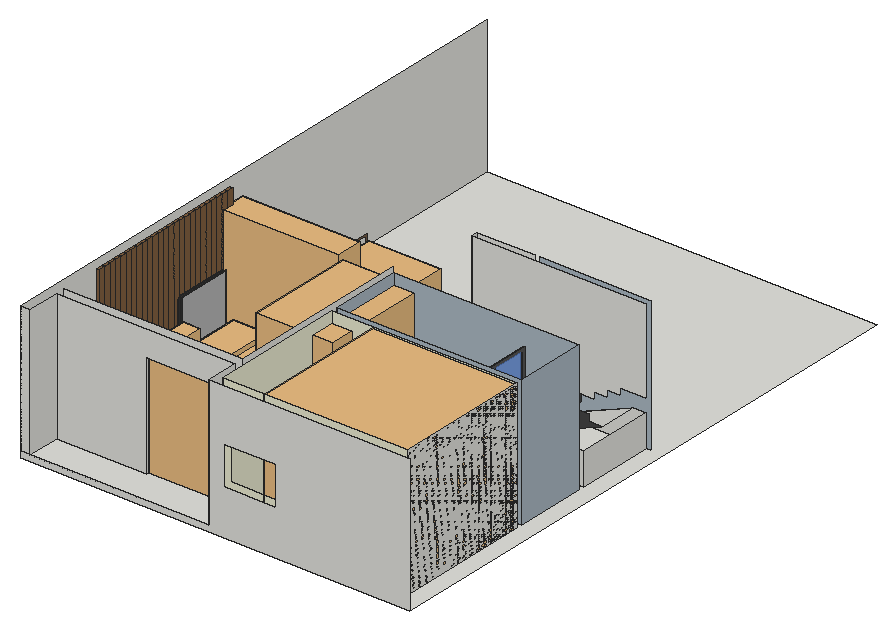
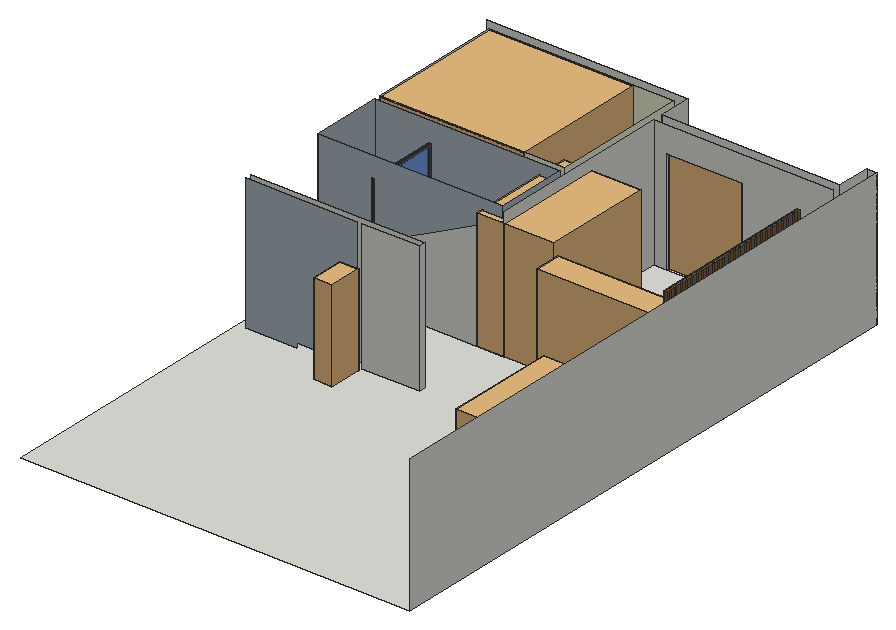
# SketchUp Ruby script. Lengths in inches.
U = 1.inch
M = Sketchup.active_model
def pt(a) = Geom::Point3d.new(a.map { |v| v * U })
def face(e, loops, mat)
  f = e.add_face(loops[0].map { |a| pt(a) })
  loops[1..].each { |l| e.add_face(l.map { |a| pt(a) }).erase! }
  f.material = f.back_material = mat if mat
  f
end
# faces: each face lists its corners as indices into pts; further lists are holes
def faces(e, pts, list, mat = nil) = list.each { |f| face(e, (f[0].is_a?(Array) ? f : [f]).map { |l| l.map { |i| pts[i] } }, mat) }
# xy, xz, yz: faces in a plane at the given z, y or x. An outline is a flat list of corners, or four numbers for a rectangle; further outlines are holes
def ring(l) = l.size == 4 ? [[l[0], l[1]], [l[2], l[1]], [l[2], l[3]], [l[0], l[3]]] : l.each_slice(2).to_a
def flat(e, list, mat, &to3) = list.each { |f| face(e, (f[0].is_a?(Array) ? f : [f]).map { |l| ring(l).map { |u, v| to3.(u, v) } }, mat) }
def xy(e, z, list, mat = nil) = flat(e, list, mat) { |x, y| [x, y, z] }
def xz(e, y, list, mat = nil) = flat(e, list, mat) { |x, z| [x, y, z] }
def yz(e, x, list, mat = nil) = flat(e, list, mat) { |y, z| [x, y, z] }
def lines(e, pts, list) = list.each { |a, b| e.add_line(pt(pts[a]), pt(pts[b])) }
# prism: a flat outline (further loops are holes) pulled along v
def prism(e, loops, v, mat = nil)
  f = face(e, loops, mat); d = Geom::Vector3d.new(v.map { |x| x * U })
  f.pushpull(f.normal.samedirection?(d) ? d.length : -d.length)
end
def box(e, o, s, mat = nil) = prism(e, [[o, [o[0] + s[0], o[1], o[2]], [o[0] + s[0], o[1] + s[1], o[2]], [o[0], o[1] + s[1], o[2]]]], [0, 0, s[2]], mat)
def at(x, y, z, deg = 0) = Geom::Transformation.translation(pt([x, y, z])) * Geom::Transformation.rotation(ORIGIN, Z_AXIS, deg.degrees)
def axes(o, x, y, z) = Geom::Transformation.new([*x, 0, *y, 0, *z, 0, *pt(o).to_a, 1])
def part(name) = M.definitions.add(name)
# library, detail: a bought-in or finely detailed component or shape, given as its bounding box
def library(name, o, s) = part(name).tap { |d| box(d.entities, o, s) }
def detail(e, o, s) = box(e.add_group.entities, o, s)
def put(e, d, t, mat = nil) = e.add_instance(d, t).tap { |i| i.material = mat if mat }
def group(e, t, mat = nil) = e.add_group.tap { |g| g.transformation = t; g.material = mat if mat }.entities
root = M.entities
M.materials.add("0746 AP 7715 LUMINOUS").color = [235, 235, 209]
M.materials.add("BRANCO").color = [255, 255, 255]
M.materials.add("Tiles Grey 04 100cm").color = [119, 132, 150]
M.materials.add("Tiles K04 100cm").color = [171, 184, 194]
M.materials.add("Tiles Marble White 03 180cm").color = [241, 241, 241]
M.materials["Tiles Marble White 03 180cm"].alpha = 0.94
M.materials.add("Wood Pecan 33-21 150cm").color = [115, 94, 72]
M.materials.add("[Color M06]").color = [86, 86, 86]
M.materials.add("[Granite Dark Gray]").color = [69, 68, 68]
M.materials.add("[Translucent Glass Blue]1").color = [100, 149, 237]
M.materials["[Translucent Glass Blue]1"].alpha = 0.5
M.materials.add("设计师SING的模型专用贴图(QQ群号：469733580) (333)25").color = [206, 205, 205]
M.materials.add("设计师SING的模型专用贴图(QQ群号：469733580) (333)26").color = [51, 51, 51]
M.materials.add("设计师SING的模型专用贴图(QQ群号：469733580) (333)27").color = [183, 183, 183]
M.materials.add("设计师SING的模型专用贴图(QQ群号：469733580) (333)28").color = [107, 107, 107]
M.materials.add("设计师SING的模型专用贴图(QQ群号：469733580) (333)6").color = [131, 97, 66]
M.materials.add("设计师SING的模型专用贴图(QQ群号：469733580) (333)8").color = [40, 40, 40]
M.materials.add("设计师SING的模型专用贴图(QQ群号：469733580) (333)9").color = [170, 158, 147]
c1 = library("main+door+wooden",[145.01,36,24],[12.59,96.04,103.74])
c2 = library("Interior+Mini+badroom_Vray",[7.09,7.875,-1.02],[132.76,181.1,119.13])
c3 = library("Door+80x210",[17.88,40.74,0],[31.52,6.14,82.69])
c4 = library("PVC+Bathroom+Door",[-64.14,19.83,292.78],[29.53,18.71,82.68])
c5 = part("Component2")
xy(c5.entities,-21.52,[[-1863.56,-2637.97,-1837.03,2637.97],[-1702.66,-2637.97,-1676.14,2637.97],[-1541.77,-2637.97,-1515.24,2637.97],[-1380.87,-2637.97,-1354.35,2637.97],[-1219.98,-2637.97,-1193.45,2637.97],
  [-1059.08,-2637.97,-1032.56,2637.97],[-898.1875,-2637.97,-871.66,2637.97],[-737.29,-2637.97,-710.77,2637.97],[-576.4,-2637.97,-549.87,2637.97],[-415.5,-2637.97,-388.97,-2637.97,-388.98,2637.97,-415.5,2637.97],
  [-254.61,-2637.97,-228.08,2637.97],[-93.71,-2637.97,-67.18,2637.97],[67.18,-2637.97,93.71,2637.97],[228.08,-2637.97,254.61,2637.97],[388.98,-2637.97,415.5,-2637.97,415.5,2637.97,388.97,2637.97],
  [549.87,-2637.97,576.4,2637.97],[710.77,-2637.97,737.29,2637.97],[871.66,-2637.97,898.1875,2637.97],[1032.56,-2637.97,1059.08,2637.97],[1193.45,-2637.97,1219.98,2637.97],
  [1354.35,-2637.97,1380.87,2637.97],[1515.24,-2637.97,1541.77,2637.97],[1676.14,-2637.97,1702.66,2637.97],[1837.03,-2637.97,1863.56,2637.97]],"设计师SING的模型专用贴图(QQ群号：469733580) (333)6")
xy(c5.entities,0,[[-2011.19,-2637.97,-1863.56,2637.97],[-1837.03,-2637.97,-1702.66,2637.97],[-1676.14,-2637.97,-1541.77,2637.97],[-1515.24,-2637.97,-1380.87,2637.97],[-1354.35,-2637.97,-1219.98,2637.97],
  [-1193.45,-2637.97,-1059.08,2637.97],[-1032.56,-2637.97,-898.1875,2637.97],[-871.66,-2637.97,-737.29,2637.97],[-710.77,-2637.97,-576.4,2637.97],[-549.87,-2637.97,-415.5,2637.97],
  [-388.97,-2637.97,-254.61,-2637.97,-254.61,2637.97,-388.98,2637.97],[-228.08,-2637.97,-93.71,2637.97],[-67.18,-2637.97,67.18,2637.97],[93.71,-2637.97,228.08,2637.97],[254.61,-2637.97,388.98,-2637.97,388.97,2637.97,254.61,2637.97],
  [415.5,-2637.97,549.87,2637.97],[576.4,-2637.97,710.77,2637.97],[737.29,-2637.97,871.66,2637.97],[898.1875,-2637.97,1032.56,2637.97],[1059.08,-2637.97,1193.45,2637.97],
  [1219.98,-2637.97,1354.35,2637.97],[1380.87,-2637.97,1515.24,2637.97],[1541.77,-2637.97,1676.14,2637.97],[1702.66,-2637.97,1837.03,2637.97],[1863.56,-2637.97,2011.19,2637.97]],"设计师SING的模型专用贴图(QQ群号：469733580) (333)6")
xz(c5.entities,-2637.97,[[-2011.19,-51.02,2011.19,0],[-1863.56,-21.52,-1837.03,0],[-1702.66,-21.52,-1676.14,0],[-1541.77,-21.52,-1515.24,0],[-1380.87,-21.52,-1354.35,0],
  [-1219.98,-21.52,-1193.45,0],[-1059.08,-21.52,-1032.56,0],[-898.1875,-21.52,-871.66,0],[-737.29,-21.52,-710.77,0],[-576.4,-21.52,-549.87,0],
  [-415.5,-21.52,-388.97,0],[-254.61,-21.52,-228.08,0],[-93.71,-21.52,-67.18,0],[67.18,-21.52,93.71,0],[228.08,-21.52,254.61,0],
  [388.98,-21.52,415.5,0],[549.87,-21.52,576.4,0],[710.77,-21.52,737.29,0],[871.66,-21.52,898.1875,0],[1032.56,-21.52,1059.08,0],
  [1193.45,-21.52,1219.98,0],[1354.35,-21.52,1380.87,0],[1515.24,-21.52,1541.77,0],[1676.14,-21.52,1702.66,0],[1837.03,-21.52,1863.56,0]],"设计师SING的模型专用贴图(QQ群号：469733580) (333)6")
xz(c5.entities,2637.97,[[-2011.19,-51.02,2011.19,0],[-1863.56,-21.52,-1837.03,0],[-1702.66,-21.52,-1676.14,0],[-1541.77,-21.52,-1515.24,0],[-1380.87,-21.52,-1354.35,0],
  [-1219.98,-21.52,-1193.45,0],[-1059.08,-21.52,-1032.56,0],[-898.1875,-21.52,-871.66,0],[-737.29,-21.52,-710.77,0],[-576.4,-21.52,-549.87,0],
  [-415.5,-21.52,-388.98,0],[-254.61,-21.52,-228.08,0],[-93.71,-21.52,-67.18,0],[67.18,-21.52,93.71,0],[228.08,-21.52,254.61,0],
  [388.97,-21.52,415.5,0],[549.87,-21.52,576.4,0],[710.77,-21.52,737.29,0],[871.66,-21.52,898.1875,0],[1032.56,-21.52,1059.08,0],
  [1193.45,-21.52,1219.98,0],[1354.35,-21.52,1380.87,0],[1515.24,-21.52,1541.77,0],[1676.14,-21.52,1702.66,0],[1837.03,-21.52,1863.56,0]],"设计师SING的模型专用贴图(QQ群号：469733580) (333)6")
yz(c5.entities,-2011.19,[[-2637.97,-51.02,2637.97,0]],"设计师SING的模型专用贴图(QQ群号：469733580) (333)6")
yz(c5.entities,-1863.56,[[-2637.97,-21.52,2637.97,0]],"设计师SING的模型专用贴图(QQ群号：469733580) (333)6")
yz(c5.entities,-1837.03,[[-2637.97,-21.52,2637.97,0]],"设计师SING的模型专用贴图(QQ群号：469733580) (333)6")
yz(c5.entities,-1702.66,[[-2637.97,-21.52,2637.97,0]],"设计师SING的模型专用贴图(QQ群号：469733580) (333)6")
yz(c5.entities,-1676.14,[[-2637.97,-21.52,2637.97,0]],"设计师SING的模型专用贴图(QQ群号：469733580) (333)6")
yz(c5.entities,-1541.77,[[-2637.97,-21.52,2637.97,0]],"设计师SING的模型专用贴图(QQ群号：469733580) (333)6")
yz(c5.entities,-1515.24,[[-2637.97,-21.52,2637.97,0]],"设计师SING的模型专用贴图(QQ群号：469733580) (333)6")
yz(c5.entities,-1380.87,[[-2637.97,-21.52,2637.97,0]],"设计师SING的模型专用贴图(QQ群号：469733580) (333)6")
yz(c5.entities,-1354.35,[[-2637.97,-21.52,2637.97,0]],"设计师SING的模型专用贴图(QQ群号：469733580) (333)6")
yz(c5.entities,-1219.98,[[-2637.97,-21.52,2637.97,0]],"设计师SING的模型专用贴图(QQ群号：469733580) (333)6")
yz(c5.entities,-1193.45,[[-2637.97,-21.52,2637.97,0]],"设计师SING的模型专用贴图(QQ群号：469733580) (333)6")
yz(c5.entities,-1059.08,[[-2637.97,-21.52,2637.97,0]],"设计师SING的模型专用贴图(QQ群号：469733580) (333)6")
yz(c5.entities,-1032.56,[[-2637.97,-21.52,2637.97,0]],"设计师SING的模型专用贴图(QQ群号：469733580) (333)6")
yz(c5.entities,-898.1875,[[-2637.97,-21.52,2637.97,0]],"设计师SING的模型专用贴图(QQ群号：469733580) (333)6")
yz(c5.entities,-871.66,[[-2637.97,-21.52,2637.97,0]],"设计师SING的模型专用贴图(QQ群号：469733580) (333)6")
yz(c5.entities,-737.29,[[-2637.97,-21.52,2637.97,0]],"设计师SING的模型专用贴图(QQ群号：469733580) (333)6")
yz(c5.entities,-710.77,[[-2637.97,-21.52,2637.97,0]],"设计师SING的模型专用贴图(QQ群号：469733580) (333)6")
yz(c5.entities,-576.4,[[-2637.97,-21.52,2637.97,0]],"设计师SING的模型专用贴图(QQ群号：469733580) (333)6")
yz(c5.entities,-549.87,[[-2637.97,-21.52,2637.97,0]],"设计师SING的模型专用贴图(QQ群号：469733580) (333)6")
yz(c5.entities,-415.5,[[-2637.97,-21.52,2637.97,0]],"设计师SING的模型专用贴图(QQ群号：469733580) (333)6")
yz(c5.entities,-254.61,[[-2637.97,-21.52,2637.97,0]],"设计师SING的模型专用贴图(QQ群号：469733580) (333)6")
yz(c5.entities,-228.08,[[-2637.97,-21.52,2637.97,0]],"设计师SING的模型专用贴图(QQ群号：469733580) (333)6")
yz(c5.entities,-93.71,[[-2637.97,-21.52,2637.97,0]],"设计师SING的模型专用贴图(QQ群号：469733580) (333)6")
yz(c5.entities,-67.18,[[-2637.97,-21.52,2637.97,0]],"设计师SING的模型专用贴图(QQ群号：469733580) (333)6")
yz(c5.entities,67.18,[[-2637.97,-21.52,2637.97,0]],"设计师SING的模型专用贴图(QQ群号：469733580) (333)6")
yz(c5.entities,93.71,[[-2637.97,-21.52,2637.97,0]],"设计师SING的模型专用贴图(QQ群号：469733580) (333)6")
yz(c5.entities,228.08,[[-2637.97,-21.52,2637.97,0]],"设计师SING的模型专用贴图(QQ群号：469733580) (333)6")
yz(c5.entities,254.61,[[-2637.97,-21.52,2637.97,0]],"设计师SING的模型专用贴图(QQ群号：469733580) (333)6")
yz(c5.entities,415.5,[[-2637.97,-21.52,2637.97,0]],"设计师SING的模型专用贴图(QQ群号：469733580) (333)6")
yz(c5.entities,549.87,[[-2637.97,-21.52,2637.97,0]],"设计师SING的模型专用贴图(QQ群号：469733580) (333)6")
yz(c5.entities,576.4,[[-2637.97,-21.52,2637.97,0]],"设计师SING的模型专用贴图(QQ群号：469733580) (333)6")
yz(c5.entities,710.77,[[-2637.97,-21.52,2637.97,0]],"设计师SING的模型专用贴图(QQ群号：469733580) (333)6")
yz(c5.entities,737.29,[[-2637.97,-21.52,2637.97,0]],"设计师SING的模型专用贴图(QQ群号：469733580) (333)6")
yz(c5.entities,871.66,[[-2637.97,-21.52,2637.97,0]],"设计师SING的模型专用贴图(QQ群号：469733580) (333)6")
yz(c5.entities,898.1875,[[-2637.97,-21.52,2637.97,0]],"设计师SING的模型专用贴图(QQ群号：469733580) (333)6")
yz(c5.entities,1032.56,[[-2637.97,-21.52,2637.97,0]],"设计师SING的模型专用贴图(QQ群号：469733580) (333)6")
yz(c5.entities,1059.08,[[-2637.97,-21.52,2637.97,0]],"设计师SING的模型专用贴图(QQ群号：469733580) (333)6")
yz(c5.entities,1193.45,[[-2637.97,-21.52,2637.97,0]],"设计师SING的模型专用贴图(QQ群号：469733580) (333)6")
yz(c5.entities,1219.98,[[-2637.97,-21.52,2637.97,0]],"设计师SING的模型专用贴图(QQ群号：469733580) (333)6")
yz(c5.entities,1354.35,[[-2637.97,-21.52,2637.97,0]],"设计师SING的模型专用贴图(QQ群号：469733580) (333)6")
yz(c5.entities,1380.87,[[-2637.97,-21.52,2637.97,0]],"设计师SING的模型专用贴图(QQ群号：469733580) (333)6")
yz(c5.entities,1515.24,[[-2637.97,-21.52,2637.97,0]],"设计师SING的模型专用贴图(QQ群号：469733580) (333)6")
yz(c5.entities,1541.77,[[-2637.97,-21.52,2637.97,0]],"设计师SING的模型专用贴图(QQ群号：469733580) (333)6")
yz(c5.entities,1676.14,[[-2637.97,-21.52,2637.97,0]],"设计师SING的模型专用贴图(QQ群号：469733580) (333)6")
yz(c5.entities,1702.66,[[-2637.97,-21.52,2637.97,0]],"设计师SING的模型专用贴图(QQ群号：469733580) (333)6")
yz(c5.entities,1837.03,[[-2637.97,-21.52,2637.97,0]],"设计师SING的模型专用贴图(QQ群号：469733580) (333)6")
yz(c5.entities,1863.56,[[-2637.97,-21.52,2637.97,0]],"设计师SING的模型专用贴图(QQ群号：469733580) (333)6")
yz(c5.entities,2011.19,[[-2637.97,-51.02,2637.97,0]],"设计师SING的模型专用贴图(QQ群号：469733580) (333)6")
p = [[-388.97,-2637.97,0],[-388.98,2637.97,0],[-388.98,2637.97,-21.52],[-388.97,-2637.97,-21.52],[388.97,2637.97,0],[388.98,-2637.97,0],
  [388.98,-2637.97,-21.52],[388.97,2637.97,-21.52]]
faces(c5.entities,p,[[0,1,2,3],[4,5,6,7]],"设计师SING的模型专用贴图(QQ群号：469733580) (333)6")
c6 = library("Component10\#1",[-136.68,-115.14,-0.07],[273.43,232.15,21.91])
c7 = part("Component8")
xy(c7.entities,51.375,[[-1109.5625,-665.28,1421.04,136.46]],"设计师SING的模型专用贴图(QQ群号：469733580) (333)25")
c8 = part("Component13\#1")
xy(c8.entities,51.375,[[-429.84,-1208.54,795.04,672.52]],"设计师SING的模型专用贴图(QQ群号：469733580) (333)27")
c9 = part("Component15\#2")
xy(c9.entities,51.375,[[69.7,-60.34,795.04,672.52]],"设计师SING的模型专用贴图(QQ群号：469733580) (333)28")
c10 = part("Component14\#1")
xy(c10.entities,0,[[-444.84,-1223.54,810.04,687.52]],"设计师SING的模型专用贴图(QQ群号：469733580) (333)26")
xy(c10.entities,61.375,[[-444.84,-1223.54,-429.84,-1208.54,-429.84,672.52,-444.84,687.52],[-444.84,-1223.54,810.04,-1223.54,795.04,-1208.54,-429.84,-1208.54],[810.04,-1223.54,810.04,687.52,795.04,672.52,795.04,-1208.54],[-429.84,672.52,795.04,672.52,810.04,687.52,-444.84,687.52]],"设计师SING的模型专用贴图(QQ群号：469733580) (333)26")
xz(c10.entities,-1223.54,[[-444.84,0,810.04,61.375]],"设计师SING的模型专用贴图(QQ群号：469733580) (333)26")
xz(c10.entities,-1208.54,[[-429.84,51.375,795.04,61.375]],"设计师SING的模型专用贴图(QQ群号：469733580) (333)26")
xz(c10.entities,672.52,[[-429.84,51.375,795.04,61.375]],"设计师SING的模型专用贴图(QQ群号：469733580) (333)26")
xz(c10.entities,687.52,[[-444.84,0,810.04,61.375]],"设计师SING的模型专用贴图(QQ群号：469733580) (333)26")
yz(c10.entities,-444.84,[[-1223.54,0,687.52,61.375]],"设计师SING的模型专用贴图(QQ群号：469733580) (333)26")
yz(c10.entities,-429.84,[[-1208.54,51.375,672.52,61.375]],"设计师SING的模型专用贴图(QQ群号：469733580) (333)26")
yz(c10.entities,795.04,[[-1208.54,51.375,672.52,61.375]],"设计师SING的模型专用贴图(QQ群号：469733580) (333)26")
yz(c10.entities,810.04,[[-1223.54,0,687.52,61.375]],"设计师SING的模型专用贴图(QQ群号：469733580) (333)26")
c11 = part("Component9")
xy(c11.entities,0,[[-1124.5625,-680.28,1436.04,151.46]],"设计师SING的模型专用贴图(QQ群号：469733580) (333)8")
xy(c11.entities,61.375,[[-1124.5625,-680.28,-1109.5625,-665.28,-1109.5625,136.46,-1124.5625,151.46],[-1124.5625,-680.28,1436.04,-680.28,1421.04,-665.28,-1109.5625,-665.28],[1436.04,-680.28,1436.04,151.46,1421.04,136.46,1421.04,-665.28],[-1109.5625,136.46,1421.04,136.46,1436.04,151.46,-1124.5625,151.46]],"设计师SING的模型专用贴图(QQ群号：469733580) (333)8")
xz(c11.entities,-680.28,[[-1124.5625,0,1436.04,61.375]],"设计师SING的模型专用贴图(QQ群号：469733580) (333)8")
xz(c11.entities,-665.28,[[-1109.5625,51.375,1421.04,61.375]],"设计师SING的模型专用贴图(QQ群号：469733580) (333)8")
xz(c11.entities,136.46,[[-1109.5625,51.375,1421.04,61.375]],"设计师SING的模型专用贴图(QQ群号：469733580) (333)8")
xz(c11.entities,151.46,[[-1124.5625,0,1436.04,61.375]],"设计师SING的模型专用贴图(QQ群号：469733580) (333)8")
yz(c11.entities,-1124.5625,[[-680.28,0,151.46,61.375]],"设计师SING的模型专用贴图(QQ群号：469733580) (333)8")
yz(c11.entities,-1109.5625,[[-665.28,51.375,136.46,61.375]],"设计师SING的模型专用贴图(QQ群号：469733580) (333)8")
yz(c11.entities,1421.04,[[-665.28,51.375,136.46,61.375]],"设计师SING的模型专用贴图(QQ群号：469733580) (333)8")
yz(c11.entities,1436.04,[[-680.28,0,151.46,61.375]],"设计师SING的模型专用贴图(QQ群号：469733580) (333)8")
c12 = part("Component16\#1")
xy(c12.entities,0,[[54.7,-75.34,810.04,687.52]],"设计师SING的模型专用贴图(QQ群号：469733580) (333)26")
xy(c12.entities,61.375,[[54.7,-75.34,69.7,-60.34,69.7,672.52,54.7,687.52],[54.7,-75.34,810.04,-75.34,795.04,-60.34,69.7,-60.34],[810.04,-75.34,810.04,687.52,795.04,672.52,795.04,-60.34],[69.7,672.52,795.04,672.52,810.04,687.52,54.7,687.52]],"设计师SING的模型专用贴图(QQ群号：469733580) (333)26")
xz(c12.entities,-75.34,[[54.7,0,810.04,61.375]],"设计师SING的模型专用贴图(QQ群号：469733580) (333)26")
xz(c12.entities,-60.34,[[69.7,51.375,795.04,61.375]],"设计师SING的模型专用贴图(QQ群号：469733580) (333)26")
xz(c12.entities,672.52,[[69.7,51.375,795.04,61.375]],"设计师SING的模型专用贴图(QQ群号：469733580) (333)26")
xz(c12.entities,687.52,[[54.7,0,810.04,61.375]],"设计师SING的模型专用贴图(QQ群号：469733580) (333)26")
yz(c12.entities,54.7,[[-75.34,0,687.52,61.375]],"设计师SING的模型专用贴图(QQ群号：469733580) (333)26")
yz(c12.entities,69.7,[[-60.34,51.375,672.52,61.375]],"设计师SING的模型专用贴图(QQ群号：469733580) (333)26")
yz(c12.entities,795.04,[[-60.34,51.375,672.52,61.375]],"设计师SING的模型专用贴图(QQ群号：469733580) (333)26")
yz(c12.entities,810.04,[[-75.34,0,687.52,61.375]],"设计师SING的模型专用贴图(QQ群号：469733580) (333)26")
c13 = library("Group81\#1",[0,0,0],[82.38,15.21,77.98])
c14 = library("Group79\#1",[-0.86,-0.19,0],[32.17,14.04,4.6])
c15 = library("Group79\#2",[0,0,0],[20.31,20.31,24.64])
c16 = library("Group79\#3",[-9.36,-9.55,0],[65.53,66.69,13.16])
c17 = library("Group80\#3",[-2.55,-2.88,-2.38],[41.24,42.9,39.42])
c18 = library("Group86\#1",[0.08,0.12,-0.78],[114.37,31.13,21.98])
c19 = library("Group95\#1",[0,0,0],[123.45,81.96,34.08])
c20 = part("bigger (29)")
put(c20.entities,c5,axes([126.625,8,103.86],[0.03937,0,0],[0,0,0.03937],[0,-0.03937,0]))
put(c20.entities,c6,axes([169.52,-83.61,24.89],[0.03601,-0.02679,0],[0.02909,0.03782,0],[0,0,0.05765]))
g1 = group(c20.entities,at(90.62,5.5,18.51))
put(g1,c7,axes([56.54,13.47,59.98],[-0.03937,0,0],[0,0,0.03937],[0,-0.03937,0]))
put(g1,c8,axes([85.33,2.42,52.34],[-0.04278,0,0],[0,0,0.04278],[0,-0.03937,0]),"设计师SING的模型专用贴图(QQ群号：469733580) (333)9")
put(g1,c9,axes([154.61,8.52,55.51],[-0.03937,0,0],[0,0,0.03937],[0,-0.03937,0]))
put(g1,c10,axes([85.33,2.42,52.34],[-0.04278,0,0],[0,0,0.04278],[0,-0.03937,0]))
put(g1,c11,axes([56.54,13.47,59.98],[-0.03937,0,0],[0,0,0.03937],[0,-0.03937,0]))
put(g1,c12,axes([154.61,8.52,55.51],[-0.03937,0,0],[0,0,0.03937],[0,-0.03937,0]))
put(c20.entities,c13,at(50.06,-18.85,-0.02))
put(c20.entities,c14,at(103.26,-89.8,13.25))
put(c20.entities,c15,at(158.66,-94.98,0.28))
put(c20.entities,c16,at(87.99,-105.98,0.18))
put(c20.entities,c17,at(27.4,-64.1875,0.22))
put(c20.entities,c18,at(75.46,-36.56,18.35))
put(c20.entities,c19,at(71.05,-83.4,0.13))
c21 = part("sofa-set-sketchup-46")
put(c21.entities,c20,at(-137.28,74.39,0))
c22 = library("1.1+TV+UNIT",[4.49,5.68,0],[132.73,70.56,110.24])
c23 = part("Group\#31")
xy(c23.entities,0,[[0,0,2,78]],"[Color M06]")
xy(c23.entities,2,[[0,2,1,39],[1.5,2,2,39],[0,39,0.5,76],[1,39,2,76]],"[Color M06]")
xy(c23.entities,2,[[1,2,1.5,39],[0.5,39,1,76]],"[Translucent Glass Blue]1")
xy(c23.entities,108.71,[[0,2,1,39],[1.5,2,2,39],[0,39,0.5,76],[1,39,2,76]],"[Color M06]")
xy(c23.entities,108.71,[[1,2,1.5,39],[0.5,39,1,76]],"[Translucent Glass Blue]1")
xy(c23.entities,110.71,[[0,0,2,78]],"[Color M06]")
xz(c23.entities,0,[[0,0,2,110.71]],"[Color M06]")
xz(c23.entities,2,[[0,2,1,108.71],[1.5,2,2,108.71]],"[Color M06]")
xz(c23.entities,2,[[1,2,1.5,108.71]],"[Translucent Glass Blue]1")
xz(c23.entities,39,[[0.5,2,1,108.71],[1,2,1.5,108.71]],"[Translucent Glass Blue]1")
xz(c23.entities,76,[[0,2,0.5,108.71],[1,2,2,108.71]],"[Color M06]")
xz(c23.entities,76,[[0.5,2,1,108.71]],"[Translucent Glass Blue]1")
xz(c23.entities,78,[[0,0,2,110.71]],"[Color M06]")
yz(c23.entities,0,[[[0,0,78,110.71],[2,2,76,108.71]]],"[Color M06]")
yz(c23.entities,0.5,[[39,2,76,108.71]],"[Translucent Glass Blue]1")
yz(c23.entities,1,[[2,2,39,108.71],[39,2,76,108.71]],"[Translucent Glass Blue]1")
yz(c23.entities,1.5,[[2,2,39,108.71]],"[Translucent Glass Blue]1")
yz(c23.entities,2,[[[0,0,78,110.71],[2,2,76,108.71]]],"[Color M06]")
c24 = library("Group\#138",[0,0,0],[13.73,23.69,16.64])
c25 = library("Group\#175",[0,0,0],[4.31,6.23,4.8])
c26 = library("PARTITION+WALL",[139.45,-12.01,0],[94.49,25.02,85.91])
c27 = library("Brutalist+modern+kitchen+and+dining+room",[-501.49,-139.75,-0.01],[151.69,99.73,55.72])
xy(root,-6,[[0,0,360,540]])
xy(root,0,[[9,0,174,0,174,30.5,162,30.5,162,39.5,92.875,39.5,92.875,30.5,9,30.5]])
xy(root,0,[[180,141,351,207]],"Tiles Grey 04 100cm")
xy(root,0,[[180,9,351,9,351,135,216,135,216,141,186,141,186,135,180,135]],"Tiles Marble White 03 180cm")
xy(root,6,[[9,242.61,28.6875,364.7]],"Wood Pecan 33-21 150cm")
xy(root,6,[[255,249,267,285]],"[Granite Dark Gray]")
xy(root,7,[[28.39,273.63,28.6875,273.93]],"Wood Pecan 33-21 150cm")
xy(root,12,[[267,249,279,285]],"[Granite Dark Gray]")
xy(root,18,[[279,249,291,285]],"[Granite Dark Gray]")
xz(root,0,[[[0,-6,360,-6,360,120,174,120,174,0,0,0],[188,36,236,72]],[0,0,9,120]])
xz(root,9,[[[180,0,351,120],[188,36,236,72]]],"0746 AP 7715 LUMINOUS")
xz(root,30.5,[[9,0,92.875,0,92.875,96,162,96,162,0,174,0,174,120,9,120]])
xz(root,39.5,[[9,0,9,120,174,120,174,0,162,0,162,96,92.875,96,92.875,0]])
xz(root,93,[[174,0,180,84]])
xz(root,129,[[174,0,180,84]])
xz(root,135,[[180,0,186,0,186,72,216,72,216,0,351,0,351,120,180,120]],"0746 AP 7715 LUMINOUS")
xz(root,141,[[180,0,180,120,351,120,351,0,216,0,216,72,186,72,186,0]],"Tiles K04 100cm")
xz(root,207,[[180,0,351,120]],"Tiles K04 100cm")
xz(root,213,[[174,0,174,112.5,327,36,327,30,351,30,351,0]])
xz(root,242.61,[[9,6,28.6875,30]],"Wood Pecan 33-21 150cm")
xz(root,249,[[255,0,267,0,339,30,327,30,327,36,315,36,315,30,303,30,303,24,291,24,291,18,279,18,279,12,267,12,267,6,255,6]],"[Granite Dark Gray]")
xz(root,273.63,[[28.39,7,28.6875,29]],"Wood Pecan 33-21 150cm")
xz(root,273.93,[[28.39,7,28.6875,29]],"Wood Pecan 33-21 150cm")
xz(root,285,[[189.8125,0,255,0,255,6,267,6,267,12,279,12,279,18,291,18,291,24,303,24,303,30,315,30,315,36,327,36,327,42,351,42,351,120,189.8125,120],[267,0,351,0,351,30,339,30]])
xz(root,291,[[189.8125,0,243,120]])
xz(root,291,[[303,-4,303,0,248,0,248,120,351,120,351,-4]],"Tiles K04 100cm")
xz(root,295,[[243,0,248,84]])
yz(root,0,[[0,-6,540,120]])
yz(root,9,[[0,0,30.5,120]])
yz(root,9,[[242.61,0,364.7,3],[242.61,3,364.7,6]],"Wood Pecan 33-21 150cm")
yz(root,28.39,[[273.63,7,273.93,29]],"Wood Pecan 33-21 150cm")
yz(root,28.6875,[[[242.61,6,364.7,30],[243.61,7,363.7,29]],[243.61,7,273.63,29],[273.93,7,303.65,29]],"Wood Pecan 33-21 150cm")
yz(root,92.875,[[30.5,0,39.5,96]])
yz(root,162,[[30.5,0,39.5,96]])
yz(root,174,[[0,0,30.5,120],[39.5,0,39.5,120,213,120,213,0,129,0,129,84,93,84,93,0]])
yz(root,180,[[9,0,93,0,93,84,129,84,129,0,135,0,135,120,9,120]],"0746 AP 7715 LUMINOUS")
yz(root,180,[[141,0,207,120]],"Tiles K04 100cm")
yz(root,186,[[135,0,141,72]],"0746 AP 7715 LUMINOUS")
yz(root,189.8125,[[285,0,291,120]])
yz(root,216,[[135,0,141,72]],"0746 AP 7715 LUMINOUS")
yz(root,255,[[249,0,285,6]],"[Granite Dark Gray]")
yz(root,267,[[249,6,285,12]],"[Granite Dark Gray]")
yz(root,279,[[249,12,285,18]],"[Granite Dark Gray]")
yz(root,291,[[249,18,285,24]],"[Granite Dark Gray]")
yz(root,351,[[9,0,135,120],[213,0,285,30]])
yz(root,351,[[141,0,207,120]],"Tiles K04 100cm")
p = [[267,285,0],[339,285,30],[339,249,30],[267,249,0],[27,234.72,0],[9,234.72,0]]
faces(root,p,[[0,1,2,3]])
lines(root,p,[[4,5]])
put(root,c1,axes([187.91,-21.11,-22.21],[0,0.37113,0],[-0.71974,0,0],[0,0,0.92536]))
put(root,c2,axes([358.09,140.48,1.02],[-1,0,0],[0,-0.69574,0],[0,0,1]),"0746 AP 7715 LUMINOUS")
put(root,c3,axes([220.08,72.58,0],[0,1.14198,0],[-1,0,0],[0,0,1.0158]))
put(root,c4,axes([251.17,119.1,-254.97],[1.016,0,0],[0,0.92,0],[0,0,0.87086]))
put(root,c21,axes([93.4,164.94,-0.9],[0,0.97215,0],[-1,0,0],[0,0,0.58207]))
put(root,c22,axes([122.66,216.41,-0.24],[0,-0.75867,0],[1,0,0],[0,0,1]))
put(root,c23,axes([299.29,141,0],[0.85,0,0],[0,0.84615,0],[0,0,0.9095]))
put(root,c24,at(266.64,186.75,0),"BRANCO")
put(root,c25,at(290.78,207,19.1,-90))
put(root,c26,axes([-151.37,232.75,0],[1.15,0,0],[0,1,0],[0,0,1.24]))
put(root,c27,axes([138.09,11.41,0],[0,-0.67,0],[0.67,0,0],[0,0,0.67]))
put(root,c4,axes([225.23,259.83,-297.47],[0,-1.016,0],[0.92,0,0],[0,0,1.016]))
